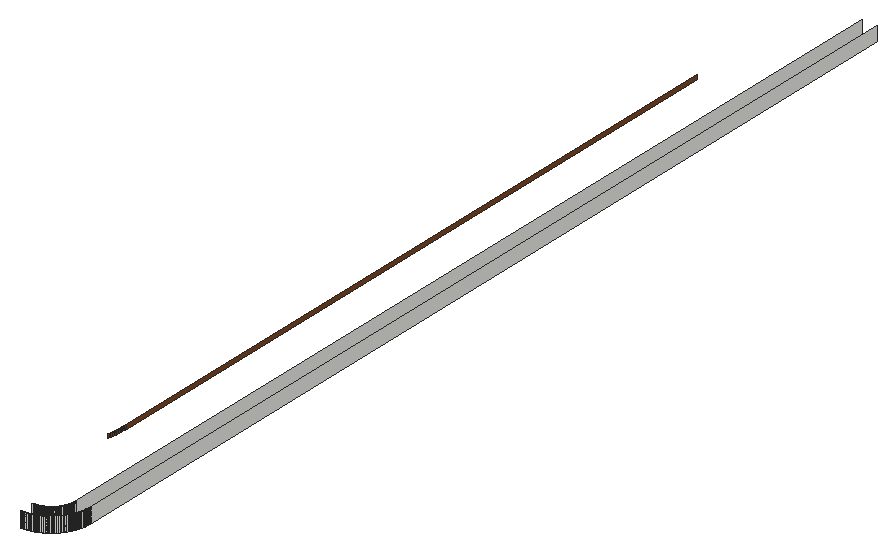
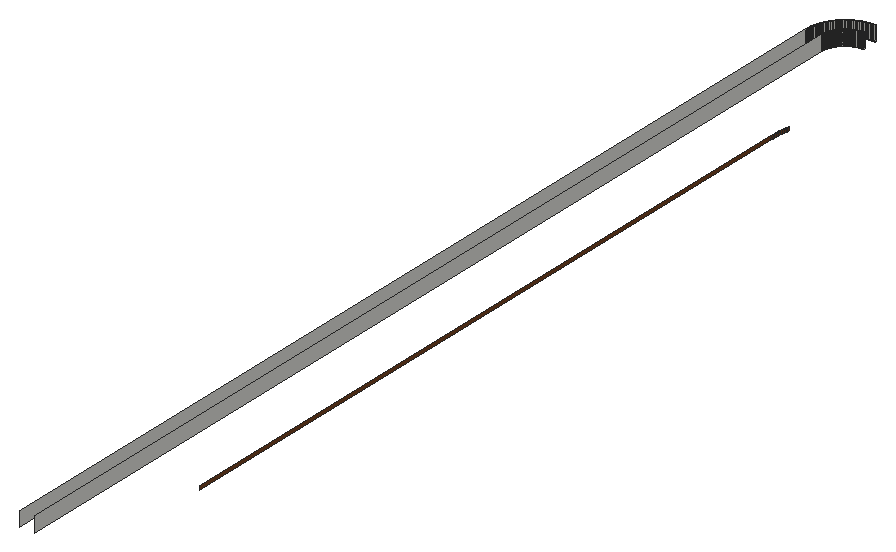
# SketchUp Ruby script. Lengths in inches.
U = 1.inch
M = Sketchup.active_model
def pt(a) = Geom::Point3d.new(a.map { |v| v * U })
def face(e, loops, mat)
  f = e.add_face(loops[0].map { |a| pt(a) })
  loops[1..].each { |l| e.add_face(l.map { |a| pt(a) }).erase! }
  f.material = f.back_material = mat if mat
  f
end
# faces: each face lists its corners as indices into pts; further lists are holes
def faces(e, pts, list, mat = nil) = list.each { |f| face(e, (f[0].is_a?(Array) ? f : [f]).map { |l| l.map { |i| pts[i] } }, mat) }
# xy, xz, yz: faces in a plane at the given z, y or x. An outline is a flat list of corners, or four numbers for a rectangle; further outlines are holes
def ring(l) = l.size == 4 ? [[l[0], l[1]], [l[2], l[1]], [l[2], l[3]], [l[0], l[3]]] : l.each_slice(2).to_a
def flat(e, list, mat, &to3) = list.each { |f| face(e, (f[0].is_a?(Array) ? f : [f]).map { |l| ring(l).map { |u, v| to3.(u, v) } }, mat) }
def xy(e, z, list, mat = nil) = flat(e, list, mat) { |x, y| [x, y, z] }
def xz(e, y, list, mat = nil) = flat(e, list, mat) { |x, z| [x, y, z] }
def yz(e, x, list, mat = nil) = flat(e, list, mat) { |y, z| [x, y, z] }
def lines(e, pts, list) = list.each { |a, b| e.add_line(pt(pts[a]), pt(pts[b])) }
# prism: a flat outline (further loops are holes) pulled along v
def prism(e, loops, v, mat = nil)
  f = face(e, loops, mat); d = Geom::Vector3d.new(v.map { |x| x * U })
  f.pushpull(f.normal.samedirection?(d) ? d.length : -d.length)
end
def box(e, o, s, mat = nil) = prism(e, [[o, [o[0] + s[0], o[1], o[2]], [o[0] + s[0], o[1] + s[1], o[2]], [o[0], o[1] + s[1], o[2]]]], [0, 0, s[2]], mat)
def at(x, y, z, deg = 0) = Geom::Transformation.translation(pt([x, y, z])) * Geom::Transformation.rotation(ORIGIN, Z_AXIS, deg.degrees)
def axes(o, x, y, z) = Geom::Transformation.new([*x, 0, *y, 0, *z, 0, *pt(o).to_a, 1])
def part(name) = M.definitions.add(name)
# library, detail: a bought-in or finely detailed component or shape, given as its bounding box
def library(name, o, s) = part(name).tap { |d| box(d.entities, o, s) }
def detail(e, o, s) = box(e.add_group.entities, o, s)
def put(e, d, t, mat = nil) = e.add_instance(d, t).tap { |i| i.material = mat if mat }
def group(e, t, mat = nil) = e.add_group.tap { |g| g.transformation = t; g.material = mat if mat }.entities
root = M.entities
M.materials.add("[Wood Veneer 01]3").color = [120, 70, 37]
xz(root,33.75,[[143.98,121,144.07,123],[144.07,121,144.14,123],[144.14,121,144.21,123]])
xz(root,33.76,[[144.27,121,144.34,123]])
xz(root,33.77,[[144.41,121,144.48,123]])
xz(root,33.8,[[144.69,121,144.75,123]])
xz(root,35.75,[[143.97,121,144.04,123],[144.04,121,144.09,123],[144.09,121,144.13,123],[144.13,121,144.17,123]])
xz(root,35.76,[[144.21,121,144.25,123],[144.25,121,144.3,123]])
xz(root,35.77,[[144.34,121,144.38,123]])
xz(root,35.78,[[144.42,121,144.47,123]])
xz(root,35.8,[[144.55,121,144.59,123]])
yz(root,139.5,[[56.65,121,56.82,121.5],[56.82,121,57,121.5],[57,121,153,121.5]],"[Wood Veneer 01]3")
yz(root,147.2,[[38.41,121,38.45,123]])
yz(root,147.22,[[38.53,121,38.58,123]])
yz(root,147.23,[[38.62,121,38.66,123]])
yz(root,147.24,[[38.7,121,38.75,123],[38.75,121,38.79,123]])
yz(root,147.25,[[38.83,121,38.87,123],[38.87,121,38.91,123],[38.91,121,38.96,123],[38.96,121,39.03,123],[39.03,121,170.97,123]])
yz(root,149.2,[[38.25,121,38.31,123]])
yz(root,149.23,[[38.52,121,38.59,123]])
yz(root,149.24,[[38.66,121,38.73,123]])
yz(root,149.25,[[38.79,121,38.86,123],[38.86,121,38.93,123],[38.93,121,39.02,123],[39.02,121,170.98,123]])
p = [[144.21,33.75,121],[144.27,33.76,121],[144.27,33.76,123],[144.21,33.75,123],[144.34,33.76,121],[144.41,33.77,121],
  [144.41,33.77,123],[144.34,33.76,123],[144.48,33.77,121],[144.55,33.78,121],[144.55,33.78,123],[144.48,33.77,123],
  [144.62,33.79,121],[144.62,33.79,123],[144.69,33.8,121],[144.69,33.8,123],[144.75,33.8,121],[144.82,33.81,121],
  [144.82,33.81,123],[144.75,33.8,123],[144.89,33.83,121],[144.89,33.83,123],[144.96,33.84,121],[144.96,33.84,123],
  [145.02,33.85,121],[145.02,33.85,123],[145.09,33.86,121],[145.09,33.86,123],[145.16,33.88,121],[145.16,33.88,123],
  [145.23,33.9,121],[145.23,33.9,123],[145.29,33.91,121],[145.29,33.91,123],[145.36,33.93,121],[145.36,33.93,123],
  [145.43,33.95,121],[145.43,33.95,123],[145.49,33.97,121],[145.49,33.97,123],[145.56,33.99,121],[145.56,33.99,123],
  [145.62,34.01,121],[145.62,34.01,123],[145.6875,34.03,121],[145.6875,34.03,123],[145.75,34.05,121],[145.75,34.05,123],
  [145.82,34.07,121],[145.82,34.07,123],[145.88,34.1,121],[145.88,34.1,123],[145.95,34.125,121],[145.95,34.125,123],
  [146.01,34.15,121],[146.01,34.15,123],[146.07,34.18,121],[146.07,34.18,123],[146.14,34.2,121],[146.14,34.2,123],
  [146.2,34.23,121],[146.2,34.23,123],[146.26,34.26,121],[146.26,34.26,123],[146.32,34.29,121],[146.32,34.29,123],
  [146.38,34.32,121],[146.38,34.32,123],[146.44,34.35,121],[146.44,34.35,123],[146.51,34.39,121],[146.51,34.39,123],
  [146.57,34.42,121],[146.57,34.42,123],[146.625,34.45,121],[146.625,34.45,123],[146.68,34.49,121],[146.68,34.49,123],
  [146.74,34.52,121],[146.74,34.52,123],[146.8,34.56,121],[146.8,34.56,123],[146.86,34.6,121],[146.86,34.6,123],
  [146.92,34.63,121],[146.92,34.63,123],[146.97,34.67,121],[146.97,34.67,123],[147.03,34.71,121],[147.03,34.71,123],
  [147.09,34.75,121],[147.09,34.75,123],[147.14,34.79,121],[147.14,34.79,123],[147.2,34.84,121],[147.2,34.84,123],
  [147.25,34.88,121],[147.25,34.88,123],[147.3,34.92,121],[147.3,34.92,123],[147.36,34.96,121],[147.36,34.96,123],
  [147.41,35.01,121],[147.41,35.01,123],[147.46,35.05,121],[147.46,35.05,123],[147.51,35.1,121],[147.51,35.1,123],
  [147.5625,35.14,121],[147.5625,35.14,123],[147.61,35.19,121],[147.61,35.19,123],[147.66,35.24,121],[147.66,35.24,123],
  [147.71,35.29,121],[147.71,35.29,123],[147.76,35.34,121],[147.76,35.34,123],[147.81,35.39,121],[147.81,35.39,123],
  [147.86,35.4375,121],[147.86,35.4375,123],[147.9,35.49,121],[147.9,35.49,123],[147.95,35.54,121],[147.95,35.54,123],
  [147.99,35.59,121],[147.99,35.59,123],[148.04,35.64,121],[148.04,35.64,123],[148.08,35.7,121],[148.08,35.7,123],
  [148.12,35.75,121],[148.12,35.75,123],[148.16,35.8,121],[148.16,35.8,123],[144.21,35.76,121],[144.17,35.75,121],
  [144.17,35.75,123],[144.21,35.76,123],[144.34,35.77,121],[144.3,35.76,121],[144.3,35.76,123],[144.34,35.77,123],
  [144.42,35.78,121],[144.38,35.77,121],[144.38,35.77,123],[144.42,35.78,123],[144.51,35.79,121],[144.47,35.78,121],
  [144.47,35.78,123],[144.51,35.79,123],[144.55,35.8,121],[144.55,35.8,123],[144.63,35.8125,121],[144.59,35.8,121],
  [144.59,35.8,123],[144.63,35.8125,123],[144.68,35.82,121],[144.68,35.82,123],[144.72,35.83,121],[144.72,35.83,123],
  [144.76,35.84,121],[144.76,35.84,123],[144.8,35.85,121],[144.8,35.85,123],[148.21,35.86,121],[148.21,35.86,123],
  [144.84,35.86,121],[144.84,35.86,123],[144.88,35.87,121],[144.88,35.87,123],[144.92,35.88,121],[144.92,35.88,123],
  [144.96,35.9,121],[144.96,35.9,123],[145,35.91,121],[145,35.91,123],[145.04,35.92,121],[145.04,35.92,123],
  [145.08,35.9375,121],[145.08,35.9375,123],[145.125,35.95,121],[145.125,35.95,123],[148.25,35.91,121],[148.25,35.91,123],
  [148.29,35.97,121],[148.29,35.97,123],[145.16,35.97,121],[145.16,35.97,123],[145.2,35.98,121],[145.2,35.98,123],
  [145.24,36,121],[145.24,36,123],[145.28,36.01,121],[145.28,36.01,123],[145.32,36.03,121],[145.32,36.03,123],
  [145.36,36.05,121],[145.36,36.05,123],[145.4,36.07,121],[145.4,36.07,123],[148.33,36.03,121],[148.33,36.03,123],
  [148.37,36.08,121],[148.37,36.08,123],[145.4375,36.09,121],[145.4375,36.09,123],[145.48,36.1,121],[145.48,36.1,123],
  [145.51,36.125,121],[145.51,36.125,123],[145.55,36.14,121],[145.55,36.14,123],[145.59,36.16,121],[145.59,36.16,123],
  [148.4,36.14,121],[148.4,36.14,123],[148.44,36.2,121],[148.44,36.2,123],[145.625,36.1875,121],[145.625,36.1875,123],
  [145.66,36.21,121],[145.66,36.21,123],[145.7,36.23,121],[145.7,36.23,123],[145.73,36.25,121],[145.73,36.25,123],
  [148.48,36.26,121],[148.48,36.26,123],[145.77,36.27,121],[145.77,36.27,123],[145.81,36.3,121],[145.81,36.3,123],
  [145.84,36.32,121],[145.84,36.32,123],[145.875,36.35,121],[145.875,36.35,123],[145.91,36.37,121],[145.91,36.37,123],
  [148.51,36.32,121],[148.51,36.32,123],[148.55,36.375,121],[148.55,36.375,123],[145.94,36.4,121],[145.94,36.4,123],
  [145.98,36.42,121],[145.98,36.42,123],[146.01,36.45,121],[146.01,36.45,123],[146.05,36.47,121],[146.05,36.47,123],
  [148.58,36.43,121],[148.58,36.43,123],[148.61,36.49,121],[148.61,36.49,123],[146.08,36.5,121],[146.08,36.5,123],
  [146.11,36.53,121],[146.11,36.53,123],[146.14,36.56,121],[146.14,36.56,123],[148.65,36.56,121],[148.65,36.56,123],
  [146.17,36.58,121],[146.17,36.58,123],[146.21,36.61,121],[146.21,36.61,123],[146.24,36.64,121],[146.24,36.64,123],
  [146.27,36.67,121],[146.27,36.67,123],[148.68,36.62,121],[148.68,36.62,123],[148.71,36.68,121],[148.71,36.68,123],
  [146.3,36.7,121],[146.3,36.7,123],[146.33,36.73,121],[146.33,36.73,123],[146.36,36.76,121],[146.36,36.76,123],
  [148.74,36.74,121],[148.74,36.74,123],[148.77,36.8,121],[148.77,36.8,123],[146.39,36.79,121],[146.39,36.79,123],
  [146.42,36.83,121],[146.42,36.83,123],[146.44,36.86,121],[146.44,36.86,123],[148.8,36.86,121],[148.8,36.86,123],
  [146.47,36.89,121],[146.47,36.89,123],[146.5,36.92,121],[146.5,36.92,123],[146.53,36.95,121],[146.53,36.95,123],
  [148.82,36.93,121],[148.82,36.93,123],[148.85,36.99,121],[148.85,36.99,123],[146.55,36.99,121],[146.55,36.99,123],
  [146.58,37.02,121],[146.58,37.02,123],[146.6,37.06,121],[146.6,37.06,123],[148.875,37.05,121],[148.875,37.05,123],
  [146.63,37.09,121],[146.63,37.09,123],[146.65,37.125,121],[146.65,37.125,123],[146.68,37.16,121],[146.68,37.16,123],
  [148.9,37.12,121],[148.9,37.12,123],[148.93,37.18,121],[148.93,37.18,123],[146.7,37.19,121],[146.7,37.19,123],
  [146.73,37.23,121],[146.73,37.23,123],[146.75,37.27,121],[146.75,37.27,123],[148.95,37.25,121],[148.95,37.25,123],
  [148.97,37.3125,121],[148.97,37.3125,123],[146.77,37.3,121],[146.77,37.3,123],[146.79,37.34,121],[146.79,37.34,123],
  [146.8125,37.375,121],[146.8125,37.375,123],[148.99,37.38,121],[148.99,37.38,123],[146.84,37.41,121],[146.84,37.41,123],
  [146.86,37.45,121],[146.86,37.45,123],[146.875,37.49,121],[146.875,37.49,123],[149.01,37.44,121],[149.01,37.44,123],
  [149.03,37.51,121],[149.03,37.51,123],[146.9,37.52,121],[146.9,37.52,123],[146.91,37.5625,121],[146.91,37.5625,123],
  [149.05,37.57,121],[149.05,37.57,123],[146.93,37.6,121],[146.93,37.6,123],[146.95,37.64,121],[146.95,37.64,123],
  [146.97,37.68,121],[146.97,37.68,123],[149.07,37.64,121],[149.07,37.64,123],[149.09,37.71,121],[149.09,37.71,123],
  [146.99,37.72,121],[146.99,37.72,123],[147,37.76,121],[147,37.76,123],[149.1,37.77,121],[149.1,37.77,123],
  [147.02,37.8,121],[147.02,37.8,123],[147.03,37.84,121],[147.03,37.84,123],[147.05,37.875,121],[147.05,37.875,123],
  [149.12,37.84,121],[149.12,37.84,123],[149.14,37.91,121],[149.14,37.91,123],[147.0625,37.92,121],[147.0625,37.92,123],
  [147.08,37.96,121],[147.08,37.96,123],[149.15,37.98,121],[149.15,37.98,123],[147.09,38,121],[147.09,38,123],
  [147.1,38.04,121],[147.1,38.04,123],[147.12,38.08,121],[147.12,38.08,123],[149.16,38.04,121],[149.16,38.04,123],
  [149.17,38.11,121],[149.17,38.11,123],[147.13,38.12,121],[147.13,38.12,123],[147.14,38.16,121],[147.14,38.16,123],
  [149.19,38.18,121],[149.19,38.18,123],[147.15,38.2,121],[147.15,38.2,123],[147.16,38.24,121],[147.16,38.24,123],
  [147.17,38.28,121],[147.17,38.28,123],[149.2,38.25,121],[149.2,38.25,123],[147.18,38.32,121],[147.18,38.32,123],
  [147.1875,38.37,121],[147.1875,38.37,123],[149.2,38.31,121],[149.21,38.38,121],[149.21,38.38,123],[149.2,38.31,123],
  [147.2,38.41,121],[147.2,38.41,123],[147.21,38.49,121],[147.2,38.45,121],[147.2,38.45,123],[147.21,38.49,123],
  [149.22,38.45,121],[149.22,38.45,123],[147.22,38.53,121],[147.22,38.53,123],[149.23,38.52,121],[149.23,38.52,123],
  [147.23,38.62,121],[147.22,38.58,121],[147.22,38.58,123],[147.23,38.62,123],[149.23,38.59,121],[149.24,38.66,121],
  [149.24,38.66,123],[149.23,38.59,123],[147.24,38.7,121],[147.23,38.66,121],[147.23,38.66,123],[147.24,38.7,123],
  [149.24,38.73,121],[149.25,38.79,121],[149.25,38.79,123],[149.24,38.73,123],[147.25,38.83,121],[147.24,38.79,121],
  [147.24,38.79,123],[147.25,38.83,123],[139.24,54.37,121],[139.27,54.54,121],[139.27,54.54,121.5],[139.24,54.37,121.5],
  [139.31,54.71,121],[139.31,54.71,121.5],[139.33,54.89,121],[139.33,54.89,121.5],[139.36,55.0625,121],[139.36,55.0625,121.5],
  [139.38,55.24,121],[139.38,55.24,121.5],[139.41,55.41,121],[139.41,55.41,121.5],[139.43,55.59,121],[139.43,55.59,121.5],
  [139.44,55.76,121],[139.44,55.76,121.5],[139.46,55.94,121],[139.46,55.94,121.5],[139.47,56.12,121],[139.47,56.12,121.5],
  [139.48,56.29,121],[139.48,56.29,121.5],[139.49,56.47,121],[139.49,56.47,121.5],[139.5,56.65,121],[139.5,56.65,121.5]]
faces(root,p,[[0,1,2,3],[4,5,6,7],[8,9,10,11],[9,12,13,10],[12,14,15,13],[16,17,18,19],[17,20,21,18],[20,22,23,21],
  [22,24,25,23],[24,26,27,25],[26,28,29,27],[28,30,31,29],[30,32,33,31],[32,34,35,33],[34,36,37,35],[36,38,39,37],
  [38,40,41,39],[40,42,43,41],[42,44,45,43],[44,46,47,45],[46,48,49,47],[48,50,51,49],[50,52,53,51],[52,54,55,53],
  [54,56,57,55],[56,58,59,57],[58,60,61,59],[60,62,63,61],[62,64,65,63],[64,66,67,65],[66,68,69,67],[68,70,71,69],
  [70,72,73,71],[72,74,75,73],[74,76,77,75],[76,78,79,77],[78,80,81,79],[80,82,83,81],[82,84,85,83],[84,86,87,85],
  [86,88,89,87],[88,90,91,89],[90,92,93,91],[92,94,95,93],[94,96,97,95],[96,98,99,97],[98,100,101,99],[100,102,103,101],
  [102,104,105,103],[104,106,107,105],[106,108,109,107],[108,110,111,109],[110,112,113,111],[112,114,115,113],[114,116,117,115],[116,118,119,117],
  [118,120,121,119],[120,122,123,121],[122,124,125,123],[124,126,127,125],[126,128,129,127],[128,130,131,129],[130,132,133,131],[132,134,135,133],
  [136,137,138,139],[140,141,142,143],[144,145,146,147],[148,149,150,151],[152,148,151,153],[154,155,156,157],[158,154,157,159],[160,158,159,161],
  [162,160,161,163],[164,162,163,165],[134,166,167,135],[168,164,165,169],[170,168,169,171],[172,170,171,173],[174,172,173,175],[176,174,175,177],
  [178,176,177,179],[180,178,179,181],[182,180,181,183],[166,184,185,167],[184,186,187,185],[188,182,183,189],[190,188,189,191],[192,190,191,193],
  [194,192,193,195],[196,194,195,197],[198,196,197,199],[200,198,199,201],[186,202,203,187],[202,204,205,203],[206,200,201,207],[208,206,207,209],
  [210,208,209,211],[212,210,211,213],[214,212,213,215],[204,216,217,205],[216,218,219,217],[220,214,215,221],[222,220,221,223],[224,222,223,225],
  [226,224,225,227],[218,228,229,219],[230,226,227,231],[232,230,231,233],[234,232,233,235],[236,234,235,237],[238,236,237,239],[228,240,241,229],
  [240,242,243,241],[244,238,239,245],[246,244,245,247],[248,246,247,249],[250,248,249,251],[242,252,253,243],[252,254,255,253],[256,250,251,257],
  [258,256,257,259],[260,258,259,261],[254,262,263,255],[264,260,261,265],[266,264,265,267],[268,266,267,269],[270,268,269,271],[262,272,273,263],
  [272,274,275,273],[276,270,271,277],[278,276,277,279],[280,278,279,281],[274,282,283,275],[282,284,285,283],[286,280,281,287],[288,286,287,289],
  [290,288,289,291],[284,292,293,285],[294,290,291,295],[296,294,295,297],[298,296,297,299],[292,300,301,293],[300,302,303,301],[304,298,299,305],
  [306,304,305,307],[308,306,307,309],[302,310,311,303],[312,308,309,313],[314,312,313,315],[316,314,315,317],[310,318,319,311],[318,320,321,319],
  [322,316,317,323],[324,322,323,325],[326,324,325,327],[320,328,329,321],[328,330,331,329],[332,326,327,333],[334,332,333,335],[336,334,335,337],
  [330,338,339,331],[340,336,337,341],[342,340,341,343],[344,342,343,345],[338,346,347,339],[346,348,349,347],[350,344,345,351],[352,350,351,353],
  [348,354,355,349],[356,352,353,357],[358,356,357,359],[360,358,359,361],[354,362,363,355],[362,364,365,363],[366,360,361,367],[368,366,367,369],
  [364,370,371,365],[372,368,369,373],[374,372,373,375],[376,374,375,377],[370,378,379,371],[378,380,381,379],[382,376,377,383],[384,382,383,385],
  [380,386,387,381],[388,384,385,389],[390,388,389,391],[392,390,391,393],[386,394,395,387],[394,396,397,395],[398,392,393,399],[400,398,399,401],
  [396,402,403,397],[404,400,401,405],[406,404,405,407],[408,406,407,409],[402,410,411,403],[412,408,409,413],[414,412,413,415],[416,417,418,419],
  [420,414,415,421],[422,423,424,425],[417,426,427,418],[428,422,425,429],[426,430,431,427],[432,433,434,435],[436,437,438,439],[440,441,442,443],
  [444,445,446,447],[448,449,450,451]])
faces(root,p,[[452,453,454,455],[453,456,457,454],[456,458,459,457],[458,460,461,459],[460,462,463,461],[462,464,465,463],[464,466,467,465],[466,468,469,467],
  [468,470,471,469],[470,472,473,471],[472,474,475,473],[474,476,477,475],[476,478,479,477]],"[Wood Veneer 01]3")
